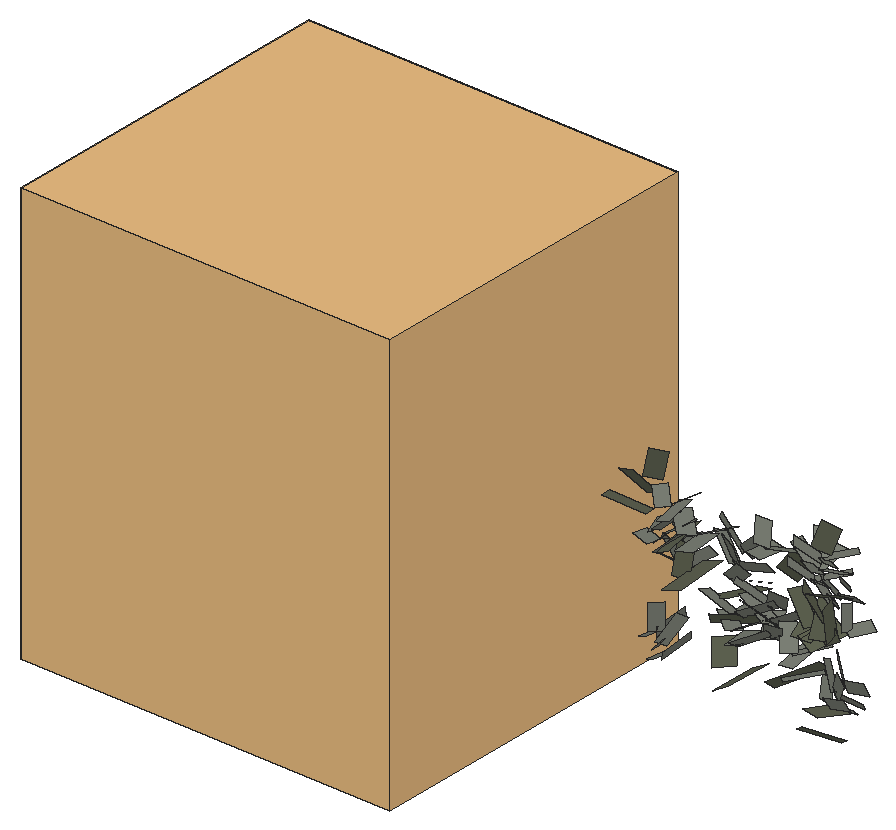
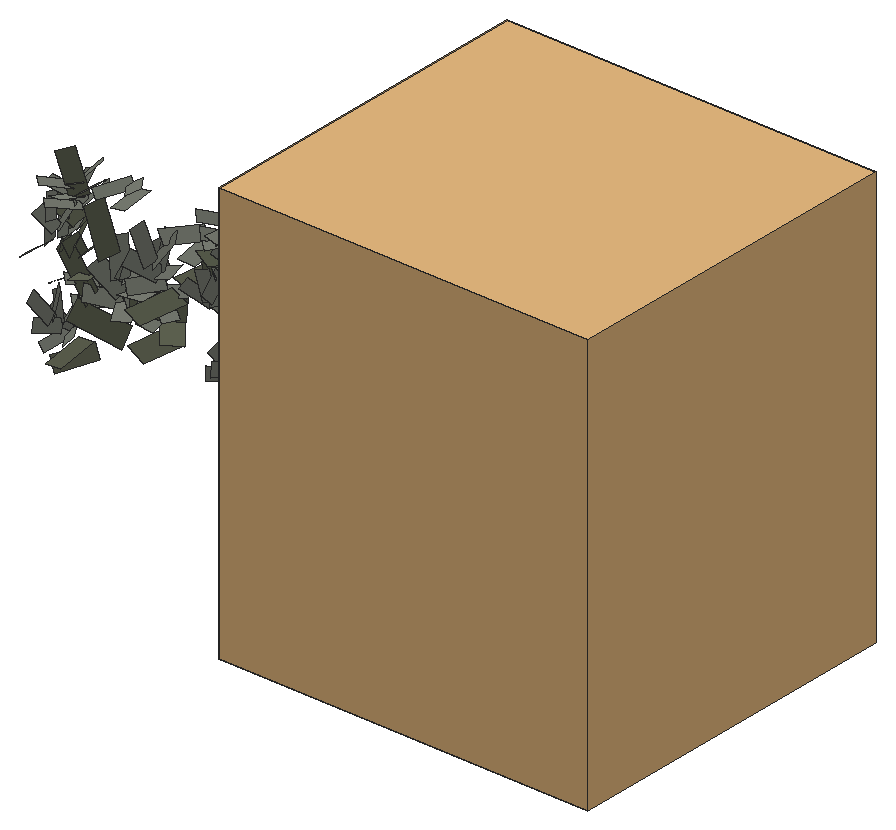
# SketchUp Ruby script. Lengths in inches.
U = 1.inch
M = Sketchup.active_model
def pt(a) = Geom::Point3d.new(a.map { |v| v * U })
def face(e, loops, mat)
  f = e.add_face(loops[0].map { |a| pt(a) })
  loops[1..].each { |l| e.add_face(l.map { |a| pt(a) }).erase! }
  f.material = f.back_material = mat if mat
  f
end
# faces: each face lists its corners as indices into pts; further lists are holes
def faces(e, pts, list, mat = nil) = list.each { |f| face(e, (f[0].is_a?(Array) ? f : [f]).map { |l| l.map { |i| pts[i] } }, mat) }
# xy, xz, yz: faces in a plane at the given z, y or x. An outline is a flat list of corners, or four numbers for a rectangle; further outlines are holes
def ring(l) = l.size == 4 ? [[l[0], l[1]], [l[2], l[1]], [l[2], l[3]], [l[0], l[3]]] : l.each_slice(2).to_a
def flat(e, list, mat, &to3) = list.each { |f| face(e, (f[0].is_a?(Array) ? f : [f]).map { |l| ring(l).map { |u, v| to3.(u, v) } }, mat) }
def xy(e, z, list, mat = nil) = flat(e, list, mat) { |x, y| [x, y, z] }
def xz(e, y, list, mat = nil) = flat(e, list, mat) { |x, z| [x, y, z] }
def yz(e, x, list, mat = nil) = flat(e, list, mat) { |y, z| [x, y, z] }
def lines(e, pts, list) = list.each { |a, b| e.add_line(pt(pts[a]), pt(pts[b])) }
# prism: a flat outline (further loops are holes) pulled along v
def prism(e, loops, v, mat = nil)
  f = face(e, loops, mat); d = Geom::Vector3d.new(v.map { |x| x * U })
  f.pushpull(f.normal.samedirection?(d) ? d.length : -d.length)
end
def box(e, o, s, mat = nil) = prism(e, [[o, [o[0] + s[0], o[1], o[2]], [o[0] + s[0], o[1] + s[1], o[2]], [o[0], o[1] + s[1], o[2]]]], [0, 0, s[2]], mat)
def at(x, y, z, deg = 0) = Geom::Transformation.translation(pt([x, y, z])) * Geom::Transformation.rotation(ORIGIN, Z_AXIS, deg.degrees)
def axes(o, x, y, z) = Geom::Transformation.new([*x, 0, *y, 0, *z, 0, *pt(o).to_a, 1])
def part(name) = M.definitions.add(name)
# library, detail: a bought-in or finely detailed component or shape, given as its bounding box
def library(name, o, s) = part(name).tap { |d| box(d.entities, o, s) }
def detail(e, o, s) = box(e.add_group.entities, o, s)
def put(e, d, t, mat = nil) = e.add_instance(d, t).tap { |i| i.material = mat if mat }
def group(e, t, mat = nil) = e.add_group.tap { |g| g.transformation = t; g.material = mat if mat }.entities
root = M.entities
M.materials.add("viburnumblaasdfas0df1w06d").color = [98, 102, 84]
M.materials.add("viburnumbladsadfasdfad0w122").color = [125, 129, 119]
c1 = part("Component\#315")
p = [[0.25,0,0],[2.05,0.01,0.35],[1.81,4.2,1.66],[0,4.19,1.3125]]
faces(c1.entities,p,[[0,1,2,3]],"viburnumbladsadfasdfad0w122")
c2 = part("viburnumblad2")
put(c2.entities,c1,axes([-19.23,-4.49,-32.18],[83.35428,0,0],[0,79.38502,0],[0,0,83.35428]))
c3 = part("Component\#314")
p = [[0.14,0,0],[2.58,0.05,0.25],[2.44,5.11,2.64],[0,5.05,2.39]]
faces(c3.entities,p,[[0,1,2,3]],"viburnumblaasdfas0df1w06d")
c4 = part("viburnumblad1\#2")
put(c4.entities,c3,axes([-37.25,6.23,19.31],[75.98784,0,0],[0,65.50676,0],[0,0,75.98784]))
c5 = library("Narrowleaf plant",[-0.44,-0.75,-1.28],[7.48,8.05,9.01])
put(root,c2,axes([1218.2,290.01,25.36],[0.00782,-0.00839,0.00329],[0.00747,0.00707,0.00029],[-0.00239,0.00208,0.01099]))
put(root,c4,axes([1220.3,287.1,19.54],[0.01555,-0.00131,0.00405],[0.00291,0.01735,-0.00577],[-0.00307,0.00585,0.01401]))
put(root,c2,axes([1216.43,292.01,11.74],[-0.00707,-0.00889,-0.00124],[0.00366,-0.00429,0.00994],[-0.0082,0.00576,0.0055]))
put(root,c2,axes([1227.36,291.17,14.07],[0.00073,-0.01105,0.00534],[0.01289,0.00219,0.00278],[-0.00345,0.00543,0.01171]))
put(root,c2,axes([1216.97,289.51,9.47],[0.00739,0.00929,0.00129],[-0.00498,0.005,-0.00749],[-0.00707,0.00455,0.00775]))
put(root,c4,axes([1226.75,287.93,11.83],[0.01166,0.00889,0.00003],[-0.00952,0.01251,-0.00648],[-0.00341,0.00442,0.01356]))
put(root,c4,axes([1226.76,287.87,9.1],[0.01294,-0.00163,0.0067],[0.00488,0.01526,-0.00571],[-0.00546,0.00626,0.01208]))
put(root,c4,axes([1215.1,290.87,25.58],[-0.00299,0.01151,-0.00453],[-0.01374,-0.0047,-0.00282],[-0.00346,0.0036,0.01051]))
put(root,c2,axes([1230.29,289.21,27.51],[0.01181,-0.00128,-0.00407],[-0.00051,0.0116,-0.00495],[0.00406,0.00486,0.00962]))
put(root,c2,axes([1216.61,291.13,21.69],[0.00162,-0.00936,0.00394],[0.00963,0.00389,0.00496],[-0.00566,0.00263,0.0077]))
put(root,c2,axes([1237.46,291.8,24.89],[-0.00706,0.00732,-0.0001],[-0.00736,-0.00703,0.00431],[0.00303,0.00306,0.01018]))
put(root,c2,axes([1238.125,292.73,25.85],[-0.01066,0.00071,0.00285],[0.00002,-0.00983,0.00251],[0.00294,0.00264,0.01033]))
put(root,c2,axes([1217.31,289.39,28.37],[0.00853,0.00755,-0.00102],[-0.0076,0.00835,-0.00179],[-0.00044,0.00202,0.01125]))
put(root,c2,axes([1237.61,292.95,24.61],[-0.00812,-0.00757,0.00318],[0.00684,-0.00722,0.00028],[0.00201,0.00231,0.01062]))
put(root,c4,axes([1218.1,288.89,22.64],[0.01125,-0.00276,0.00479],[0.00395,0.01395,-0.00123],[-0.00436,0.00225,0.01154]))
put(root,c2,axes([1231.62,293.42,15.27],[-0.01116,-0.00699,0.00046],[0.007,-0.01076,0.00634],[-0.00299,0.00562,0.01283]))
put(root,c2,axes([1231.625,292.99,17.15],[-0.01381,0.0032,-0.00202],[-0.0038,-0.01243,0.00635],[-0.00034,0.00659,0.01271]))
put(root,c2,axes([1231.18,289.32,28.89],[0.00765,0.00673,-0.00714],[-0.0085,0.00924,-0.00029],[0.00504,0.00514,0.00906]))
put(root,c2,axes([1231.3125,290.64,28.06],[0.00905,-0.00854,0.00139],[0.00807,0.00744,-0.006],[0.00301,0.00536,0.00976]))
put(root,c2,axes([1215.6,289.99,22.99],[0.00555,0.00919,-0.00035],[-0.00852,0.00498,-0.00446],[-0.00353,0.00247,0.00881]))
put(root,c2,axes([1217.5,289.58,26.8],[0.01133,-0.00035,0.0015],[0.00059,0.01187,-0.00167],[-0.00144,0.00165,0.01122]))
put(root,c2,axes([1217.64,290.75,28.04],[0.00749,-0.00804,0.00315],[0.0083,0.00786,0.00032],[-0.00239,0.00208,0.01099]))
put(root,c2,axes([1233.77,290.6,12.62],[0.00841,-0.00866,0.00086],[0.00975,0.00926,-0.00213],[0.0008,0.00201,0.01242]))
put(root,c2,axes([1226.64,290.69,18.03],[-0.00041,0.01136,-0.00703],[-0.01336,-0.0005,-0.00003],[-0.00029,0.00703,0.01137]))
put(root,c2,axes([1238.05,292.15,27.45],[-0.0073,0.00825,0.00099],[-0.00736,-0.00703,0.00431],[0.00384,0.00219,0.01013]))
put(root,c4,axes([1215.02,292.81,27.11],[-0.01098,0.00138,-0.00403],[-0.00375,-0.01153,0.00597],[-0.00261,0.00614,0.00861]))
put(root,c2,axes([1220.57,289.32,26.37],[0.0095,0.00972,-0.00486],[-0.01098,0.00941,-0.00264],[0.00181,0.00573,0.01291]))
put(root,c2,axes([1220.42,289.13,24.42],[0.01458,0.00076,-0.00047],[-0.00114,0.0144,-0.00508],[0.00059,0.00521,0.01318]))
put(root,c2,axes([1216.96,291.66,10.13],[-0.00173,-0.0098,0.00563],[0.00735,0.00343,0.00822],[-0.00865,0.00481,0.00572]))
put(root,c2,axes([1238.32,293.49,27.2],[-0.00778,-0.00725,0.00304],[0.0076,-0.00802,0.00031],[0.00201,0.00231,0.01062]))
put(root,c4,axes([1219.66,291.74,18.45],[-0.01138,-0.00264,0.00129],[0.00289,-0.0057,0.01174],[-0.00153,0.01008,0.00426]))
put(root,c4,axes([1239.28,291.54,17.94],[-0.00255,0.011,0.00125],[-0.00551,-0.00279,0.01135],[0.00975,0.00148,0.00412]))
put(root,c2,axes([1217.21,290.63,9.01],[0.00508,-0.00494,0.00777],[0.00608,0.00946,0.00204],[-0.00795,0.00351,0.00743]))
put(root,c2,axes([1215.65,292.17,23.74],[0.00169,-0.00975,0.0041],[0.00892,0.0036,0.00459],[-0.00566,0.00263,0.0077]))
put(root,c4,axes([1236.53,293.05,21.99],[-0.00267,-0.01088,0.00464],[0.01349,-0.00382,-0.00119],[0.00218,0.00422,0.01116]))
put(root,c2,axes([1215.05,290.6,11.24],[0.00707,0.00889,0.00124],[-0.00553,0.00556,-0.00832],[-0.00707,0.00455,0.00775]))
put(root,c2,axes([1215.99,290.39,9.9375],[0.00828,0.00278,0.00738],[0.00071,0.00951,-0.00438],[-0.00785,0.00396,0.00731]))
put(root,c2,axes([1220.74,290.95,25.5625],[0.01112,-0.00864,0.0042],[0.00948,0.01048,-0.0033],[-0.0007,0.0056,0.01299]))
put(root,c2,axes([1226.28,290.25,14.33],[0.0138,0.00142,0.00148],[-0.00058,0.0109,-0.00504],[-0.00186,0.00548,0.01205]))
put(root,c2,axes([1226.36,290.16,16.27],[0.00906,0.00899,-0.00397],[-0.01029,0.00825,-0.00478],[-0.00073,0.006,0.01192]))
put(root,c4,axes([1237.78,292.55,19.57],[-0.00734,0.00868,0.00063],[-0.0075,-0.00708,0.00798],[0.0058,0.00404,0.00785]))
put(root,c2,axes([1233.98,290.23,15.97],[0.00886,0.00826,-0.00347],[-0.00846,0.00932,0.00058],[0.00295,0.00192,0.0121]))
put(root,c2,axes([1225.35,293.93,19.77],[-0.00947,-0.00564,0.00547],[0.00849,-0.00835,0.00609],[0.00092,0.00846,0.01032]))
put(root,c2,axes([1231.36,294.5,18.51],[-0.01238,-0.00695,0.00189],[0.007,-0.01076,0.00634],[-0.00166,0.00641,0.0127]))
put(root,c2,axes([1233.6,290.51,14.29],[0.01246,-0.00054,-0.00182],[0.00031,0.0125,-0.00159],[0.00187,0.00153,0.01237]))
put(root,c2,axes([1226.97,292.73,16.83],[0.00041,-0.01136,0.00703],[0.01289,0.00219,0.00278],[-0.00352,0.00669,0.01102]))
put(root,c2,axes([1215.57,291.29,22.54],[0.00794,-0.00459,0.00546],[0.00496,0.0095,0.00066],[-0.00518,0.00191,0.00818]))
put(root,c2,axes([1234.26,291.74,15.55],[0.00876,-0.00902,0.0009],[0.00903,0.00857,-0.00197],[0.0008,0.00201,0.01242]))
put(root,c2,axes([1237.03,291.72,26.3125],[0.00034,0.01095,-0.00145],[-0.01033,0.00087,0.00416],[0.0042,0.00122,0.01016]))
put(root,c2,axes([1226.1875,291.47,15.41],[0.00964,-0.00707,0.00598],[0.00804,0.00897,-0.00235],[-0.00301,0.00576,0.01168]))
put(root,c4,axes([1223.01,291.42,14.85],[0.00481,-0.00968,0.00992],[0.01607,0.00349,-0.00438],[0.00046,0.01061,0.01012]))
put(root,c4,axes([1235.03,291.37,5.98],[0.00779,-0.00697,0.00615],[0.01029,0.00367,-0.00887],[0.00279,0.00941,0.00713]))
put(root,c2,axes([1218.71,293.36,20.15],[-0.01027,-0.00067,-0.00437],[-0.0029,-0.0054,0.00727],[-0.00275,0.0086,0.00434]))
put(root,c4,axes([1236.35,291.41,18.68],[0.00125,0.01083,-0.00332],[-0.01199,0.00283,0.0046],[0.00457,0.00236,0.00909]))
put(root,c2,axes([1237.2,293.64,26.01],[-0.00034,-0.01095,0.00145],[0.01148,-0.00057,-0.00162],[0.0016,0.00139,0.01085]))
put(root,c2,axes([1230.6,292.95,19.05],[-0.00715,0.01146,-0.00475],[-0.01239,-0.00628,0.0035],[0.00072,0.00585,0.01305]))
put(root,c2,axes([1238.21,293.92,8.81],[-0.00478,-0.00491,0.00751],[0.00915,-0.00588,0.00198],[0.00339,0.00769,0.00718]))
put(root,c2,axes([1214.79,291.125,23.66],[0.00954,0.00326,0.00362],[-0.00223,0.01005,-0.00307],[-0.00429,0.00184,0.00864]))
put(root,c2,axes([1225.92,294.03,21.47],[-0.01295,0.00298,0.00152],[-0.00101,-0.00935,0.0097],[0.0032,0.00918,0.00919]))
put(root,c4,axes([1237.28,291.09,17.88],[0.00373,0.00907,-0.00579],[-0.00694,0.00792,0.00773],[0.00862,0.00055,0.00603]))
put(root,c2,axes([1238.69,294.5,21.06],[-0.00905,-0.00157,0.00381],[0.00376,-0.00932,0.00479],[0.00255,0.00548,0.00745]))
put(root,c5,axes([1192.66,271.49,1.02],[0.15731,6.43674,0],[-6.43674,0.15731,0],[0,0,6.43866]))
put(root,c2,axes([1215.44,291.88,10.7],[0.00463,-0.00496,0.0092],[0.00608,0.00946,0.00204],[-0.0085,0.00407,0.00647]))
put(root,c4,axes([1231.03,292.38,8.96],[0.00205,-0.01309,0.00844],[0.0176,0.00417,0.0022],[-0.00351,0.00791,0.01312]))
put(root,c2,axes([1239.2,294.15,9.89],[-0.00948,0.00167,0.00544],[0.00331,-0.00711,0.00795],[0.00466,0.00836,0.00554]))
put(root,c4,axes([1237.07,293.57,25.73],[-0.01099,-0.00588,0.00409],[0.00754,-0.00587,0.01184],[-0.00299,0.01058,0.00715]))
put(root,c2,axes([1230.62,294.6,16.4375],[-0.0037,-0.01302,0.00469],[0.0125,-0.00235,0.00334],[-0.00247,0.0054,0.01303]))
put(root,c2,axes([1217.66,292.9,20.34],[0.0028,0.00563,-0.00742],[-0.01015,0.00031,-0.00351],[-0.00158,0.00853,0.00492]))
put(root,c2,axes([1240.85,292.46,19.58],[-0.00065,0.00993,-0.00423],[-0.00522,0.0028,0.00703],[0.00831,0.00266,0.0042]))
put(root,c4,axes([1213.88,294.47,27.8],[-0.00937,-0.00701,0.00111],[0.00657,-0.00694,0.00934],[-0.00422,0.00731,0.00713]))
put(root,c4,axes([1233.91,294.54,14.11],[-0.01053,-0.00014,0.0139],[0.01206,-0.01352,0.00899],[0.00923,0.01297,0.00712]))
put(root,c2,axes([1239.1,294.43,22.3],[-0.00889,0.00537,0.00033],[-0.00425,-0.00744,0.00652],[0.00347,0.00529,0.00723]))
put(root,c2,axes([1236.25,293.15,24.93],[0.00701,-0.00792,-0.00095],[0.00872,0.00794,-0.00187],[0.00195,0.00042,0.01087]))
put(root,c2,axes([1218.14,294.02,20.99],[-0.00494,0.0045,-0.00826],[-0.00853,-0.00405,0.00272],[-0.002,0.0084,0.00497]))
put(root,c2,axes([1229.92,292.33,17.3],[0.0037,0.01302,-0.00469],[-0.01381,0.00379,-0.00038],[0.0009,0.00462,0.01353]))
put(root,c2,axes([1225.64,291.76,17.2],[0.01322,0.00136,0.00142],[-0.00064,0.01212,-0.00561],[-0.00186,0.00548,0.01205]))
put(root,c2,axes([1218.19,293.96,19.07],[-0.00274,-0.00672,0.00719],[0.01014,0.00172,0.00518],[-0.00429,0.00766,0.00474]))
put(root,c2,axes([1239.7,295.42,23.05],[-0.00943,-0.00164,0.00397],[0.00349,-0.00863,0.00444],[0.00255,0.00548,0.00745]))
put(root,c4,axes([1234.7,291.32,16.98],[0.01142,0.00359,-0.00296],[-0.00486,0.01317,-0.00274],[0.00185,0.00298,0.01066]))
put(root,c2,axes([1218.38,294.84,20.08],[-0.00898,-0.00541,0.00233],[0.00475,-0.00369,0.00928],[-0.0037,0.00829,0.00425]))
put(root,c4,axes([1235.14,291.65,16.96],[0.00961,-0.00181,-0.00747],[-0.00022,0.01383,-0.00363],[0.00726,0.00235,0.00826]))
put(root,c2,axes([1238.04,293.59,21.76],[-0.00329,0.00963,-0.00365],[-0.0081,-0.00098,0.00442],[0.00408,0.00455,0.00739]))
put(root,c2,axes([1236.73,292.47,27.77],[0.00778,0.00725,-0.00304],[-0.00689,0.00834,0.00227],[0.00379,0.0003,0.01038]))
put(root,c2,axes([1230.2,293.89,14.89],[0.00747,-0.01197,0.00496],[0.01097,0.00676,-0.00022],[-0.0023,0.00416,0.01351]))
put(root,c4,axes([1231.26,295.67,20.91],[-0.01185,-0.00554,0.00715],[0.01005,-0.01197,0.00738],[0.00259,0.00922,0.01142]))
put(root,c2,axes([1226.03,295.75,22.3125],[-0.01014,-0.00518,0.00703],[0.00849,-0.00835,0.00609],[0.00203,0.00907,0.00962]))
put(root,c2,axes([1238.84,295.5,21.89],[-0.00444,-0.00768,0.00528],[0.00919,-0.00479,0.00064],[0.00185,0.00501,0.00791]))
put(root,c2,axes([1237.01,293.82,27.53],[0.0073,-0.00825,-0.00099],[0.00807,0.00735,-0.00173],[0.00195,0.00042,0.01087]))
put(root,c2,axes([1236.26,292.9,26.38],[0.01066,-0.00071,-0.00285],[0.00069,0.01103,-0.00015],[0.00286,-0.00003,0.01068]))
put(root,c2,axes([1224.76,295.33,20.75],[-0.00139,-0.01031,0.00841],[0.01214,-0.00182,-0.00024],[0.00145,0.00829,0.0104]))
put(root,c4,axes([1235.59,292.06,8.06],[0.01169,-0.00232,-0.00224],[0.00035,0.01065,-0.00919],[0.00321,0.00758,0.00891]))
put(root,c2,axes([1239.42,295.625,10.43],[-0.0048,-0.00448,0.0089],[0.00915,-0.00588,0.00198],[0.00393,0.00822,0.00626]))
put(root,c2,axes([1218.11,295.4,21.4],[-0.00984,-0.00064,-0.00419],[-0.00322,-0.006,0.00808],[-0.00275,0.0086,0.00434]))
put(root,c2,axes([1237.125,294.14,9.24],[0.00898,-0.00714,0.00125],[0.00484,0.00482,-0.00724],[0.0044,0.00684,0.00749]))
put(root,c2,axes([1237.97,295.09,9.7],[0.00269,-0.008,0.00714],[0.0092,-0.00069,-0.00424],[0.00383,0.00759,0.00707]))
put(root,c2,axes([1225.58,294.53,23.39],[-0.00818,0.0094,-0.00487],[-0.00969,-0.00417,0.00823],[0.00426,0.00856,0.00935]))
put(root,c2,axes([1223.96,294.32,19.74],[0.00854,-0.00981,0.00509],[0.00939,0.0055,-0.00515],[0.00179,0.0073,0.01107]))
put(root,c2,axes([1239.55,294.66,11.4375],[-0.0086,0.00684,-0.0012],[-0.00415,-0.00354,0.00962],[0.00557,0.00793,0.00532]))
put(root,c2,axes([1238.43,293.72,11],[-0.00269,0.008,-0.00714],[-0.00879,0.00257,0.00619],[0.00614,0.00718,0.00574]))
put(root,c2,axes([1229.59,292.25,15.42],[0.01189,0.00667,-0.00181],[-0.00777,0.01295,-0.00333],[0.00008,0.00361,0.01386]))
put(root,c2,axes([1240.4,293.47,19.76],[0.00544,-0.00271,-0.00718],[0.0003,0.00981,-0.00339],[0.00825,0.00152,0.00476]))
put(root,c2,axes([1237.35,293.12,10.1875],[0.00461,0.0043,-0.00854],[-0.00856,0.00831,-0.00043],[0.00603,0.00655,0.00655]))
put(root,c4,axes([1222.66,292.07,17.48],[0.01373,-0.0042,0.00303],[0.00601,0.01319,-0.00893],[-0.00014,0.00827,0.01212]))
put(root,c2,axes([1224.48,293.56,22.27],[0.00139,0.01031,-0.00841],[-0.01248,0.00393,0.00276],[0.0046,0.00756,0.01003]))
